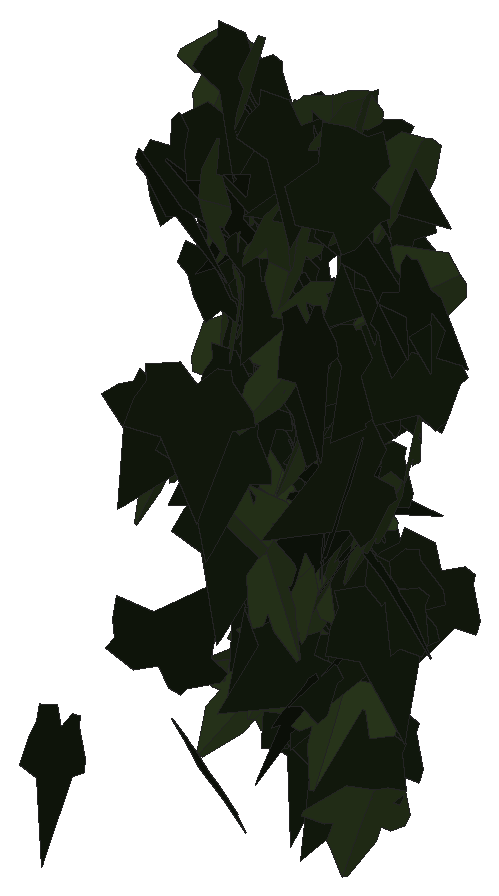
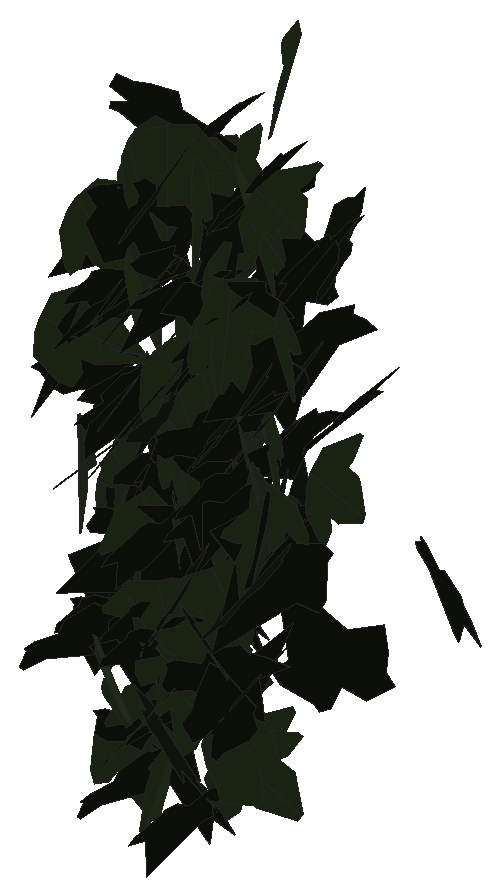
# SketchUp Ruby script. Lengths in inches.
U = 1.inch
M = Sketchup.active_model
def pt(a) = Geom::Point3d.new(a.map { |v| v * U })
def face(e, loops, mat)
  f = e.add_face(loops[0].map { |a| pt(a) })
  loops[1..].each { |l| e.add_face(l.map { |a| pt(a) }).erase! }
  f.material = f.back_material = mat if mat
  f
end
# faces: each face lists its corners as indices into pts; further lists are holes
def faces(e, pts, list, mat = nil) = list.each { |f| face(e, (f[0].is_a?(Array) ? f : [f]).map { |l| l.map { |i| pts[i] } }, mat) }
# xy, xz, yz: faces in a plane at the given z, y or x. An outline is a flat list of corners, or four numbers for a rectangle; further outlines are holes
def ring(l) = l.size == 4 ? [[l[0], l[1]], [l[2], l[1]], [l[2], l[3]], [l[0], l[3]]] : l.each_slice(2).to_a
def flat(e, list, mat, &to3) = list.each { |f| face(e, (f[0].is_a?(Array) ? f : [f]).map { |l| ring(l).map { |u, v| to3.(u, v) } }, mat) }
def xy(e, z, list, mat = nil) = flat(e, list, mat) { |x, y| [x, y, z] }
def xz(e, y, list, mat = nil) = flat(e, list, mat) { |x, z| [x, y, z] }
def yz(e, x, list, mat = nil) = flat(e, list, mat) { |y, z| [x, y, z] }
def lines(e, pts, list) = list.each { |a, b| e.add_line(pt(pts[a]), pt(pts[b])) }
# prism: a flat outline (further loops are holes) pulled along v
def prism(e, loops, v, mat = nil)
  f = face(e, loops, mat); d = Geom::Vector3d.new(v.map { |x| x * U })
  f.pushpull(f.normal.samedirection?(d) ? d.length : -d.length)
end
def box(e, o, s, mat = nil) = prism(e, [[o, [o[0] + s[0], o[1], o[2]], [o[0] + s[0], o[1] + s[1], o[2]], [o[0], o[1] + s[1], o[2]]]], [0, 0, s[2]], mat)
def at(x, y, z, deg = 0) = Geom::Transformation.translation(pt([x, y, z])) * Geom::Transformation.rotation(ORIGIN, Z_AXIS, deg.degrees)
def axes(o, x, y, z) = Geom::Transformation.new([*x, 0, *y, 0, *z, 0, *pt(o).to_a, 1])
def part(name) = M.definitions.add(name)
# library, detail: a bought-in or finely detailed component or shape, given as its bounding box
def library(name, o, s) = part(name).tap { |d| box(d.entities, o, s) }
def detail(e, o, s) = box(e.add_group.entities, o, s)
def put(e, d, t, mat = nil) = e.add_instance(d, t).tap { |i| i.material = mat if mat }
def group(e, t, mat = nil) = e.add_group.tap { |g| g.transformation = t; g.material = mat if mat }.entities
root = M.entities
M.materials.add("efeu1").color = [18, 25, 13]
M.materials.add("efeu2").color = [43, 57, 29]
c1 = part("ivyleaf_9")
p = [[1.54,2.16,1.25],[1.36,2.04,1.19],[-0.21,0.99,0.68],[-0.71,1.11,0.82],[-0.85,0.86,0.67],[-0.8,0.17,0.21],
  [-0.9,-0.01,0.1],[-0.67,-0.16,-0.02],[-0.08,-0.08,-0.05],[-0.03,-0.6,-0.4],[0.65,-0.88,-0.66],[0.83,-0.6,-0.49],
  [1.29,-0.42,-0.43],[1.8125,-0.07,-0.26],[1.21,0.44,0.15]]
faces(c1.entities,p,[[0,1,2,3,4,5,6,7,8,9,10,11,12,13,14]],"efeu1")
c2 = part("ivyleaf_10")
p = [[0,0.5,-0.03],[-0.0625,2.02,-0.43],[-0.19,2.01,-0.46],[-0.54,1.05,-0.29],[-0.52,0.625,-0.18],[-0.83,0.76,-0.28],
  [-1.16,0.64,-0.33],[-1.15,0.33,-0.24],[-0.77,-0.39,0.02],[-0.3,-0.51,0.16],[0.04,-0.48,0.23],[-0.02,2.01,-0.4375],
  [-0.06,2.01,-0.43],[0.04,-0.49,0.23],[0.67,-0.49,0.14],[1.38,0.36,-0.2],[1.375,0.51,-0.24],[0.81,0.65,-0.19],
  [0.62,0.59,-0.15],[0.6,1.09,-0.28],[0.5,1.23,-0.31]]
faces(c2.entities,p,[[0,1,2,3,4,5,6,7,8,9,10],[11,12,0,13,14,15,16,17,18,19,20]],"efeu2")
put(root,c1,axes([33.67,221.12,240.87],[0.24881,-0.31359,-0.29959],[-0.11159,0.28747,-0.39359],[0.41909,0.26272,0.07306]))
put(root,c2,axes([33.84,221.94,241.72],[-0.14855,-0.34133,0.3338],[0.13113,-0.36531,-0.3152],[0.45906,-0.0061,0.19806]))
put(root,c1,axes([33.71,221.62,239.37],[0.33206,-0.2948,-0.22985],[-0.12761,0.19957,-0.44032],[0.35136,0.35109,0.0573]))
put(root,c2,axes([33.86,221.83,237.71],[0.02125,0.46143,0.19138],[-0.03249,0.19243,-0.46034],[-0.49849,0.00713,0.03816]))
put(root,c1,axes([33.8,221.57,237.23],[0.3517,0.34567,0.0826],[0.0606,0.05617,-0.49312],[-0.3502,0.35687,-0.00239]))
put(root,c2,axes([33.73,222.03,238.11],[0.4631,-0.07129,0.17451],[0.17295,-0.02344,-0.46855],[0.07499,0.49434,0.00295]))
put(root,c1,axes([34.03,221.78,237.21],[-0.03521,-0.25322,0.4297],[0.05923,0.4256,0.25565],[-0.49523,0.0689,0.00003]))
put(root,c1,axes([33.69,220.79,240.79],[0.39813,-0.29674,-0.05863],[-0.04686,0.03523,-0.49655],[0.29882,0.40088,0.00024]))
put(root,c2,axes([34.01,221.74,238.85],[0.3219,-0.34092,-0.17364],[-0.07662,0.16488,-0.46577],[0.37485,0.32647,0.05391]))
put(root,c1,axes([33.95,221.53,239.51],[0.13311,0.29585,0.38047],[0.14222,0.35302,-0.32427],[-0.46049,0.19455,0.00983]))
put(root,c2,axes([34.02,221.64,240.13],[0.39959,-0.27835,-0.11337],[-0.07661,0.08805,-0.48619],[0.29062,0.40592,0.02772]))
put(root,c1,axes([33.78,222.41,236.97],[0.08675,-0.46042,0.17462],[0.09826,-0.15755,-0.46424],[0.48251,0.11486,0.06315]))
put(root,c2,axes([34.09,222.25,240.49],[-0.09036,-0.46837,-0.14987],[0.03951,0.14498,-0.47689],[0.49018,-0.09802,0.01081]))
put(root,c2,axes([34.34,221.37,240.95],[-0.02494,0.0348,-0.49816],[-0.30843,0.39121,0.04276],[0.39275,0.30943,0.00195]))
put(root,c2,axes([34.13,222.37,240.24],[-0.10915,-0.48793,0.00331],[-0.00759,-0.00169,-0.49994],[0.48788,-0.10919,-0.00703]))
put(root,c2,axes([34.1,222.04,238.9375],[0.24128,-0.4351,-0.04975],[-0.01733,0.04727,-0.49746],[0.43759,0.24178,0.00773]))
put(root,c2,axes([34.04,220.7,237.56],[0.04288,-0.34592,0.35847],[0.11089,-0.34414,-0.34536],[0.48566,0.10912,0.04721]))
put(root,c1,axes([33.85,222.53,239.25],[0.14288,-0.45493,0.1504],[0.05765,-0.13948,-0.47668],[0.47567,0.15356,0.0126]))
put(root,c1,axes([33.97,222.36,239],[0.00277,-0.49786,0.04616],[0.00535,-0.04612,-0.49784],[0.49996,0.00325,0.00508]))
put(root,c1,axes([34.16,221.68,236.9],[-0.18754,-0.24831,0.39137],[-0.06091,-0.40532,-0.28636],[0.45947,-0.15509,0.12178]))
put(root,c1,axes([34.25,222.34,235.14],[0.02189,0.02652,0.49882],[-0.30477,-0.39489,0.03437],[0.39578,-0.30555,-0.00112]))
put(root,c1,axes([33.91,221.24,240.2],[0.48453,0.02298,-0.12125],[0.1157,0.08626,0.47872],[0.04291,-0.49197,0.07827]))
put(root,c1,axes([34.08,222.31,238.35],[0.06115,-0.471,-0.15626],[-0.03451,0.15302,-0.47476],[0.49505,0.06885,-0.01379]))
put(root,c1,axes([34.125,221.94,241.75],[-0.0174,-0.47626,0.15125],[0.00198,-0.1514,-0.47652],[0.49969,-0.01598,0.00715]))
put(root,c1,axes([34.32,222.42,235.94],[-0.35277,-0.35374,-0.02045],[0.01422,0.01471,-0.49958],[0.35405,-0.35306,-0.00031]))
put(root,c1,axes([34.08,220.38,234.92],[-0.2088,-0.06429,0.44975],[0.43968,-0.15321,0.18222],[0.11438,0.47159,0.12051]))
put(root,c2,axes([34.42,221.91,234.4375],[-0.12256,-0.10711,-0.47276],[-0.17786,-0.44369,0.14664],[-0.45094,0.20412,0.07066]))
put(root,c1,axes([34.25,220.24,238.06],[-0.12636,-0.39607,0.27779],[0.00685,-0.28854,-0.40829],[0.48372,-0.09938,0.07834]))
put(root,c2,axes([34.23,221.83,241.89],[0.23145,-0.33891,0.2856],[0.16877,-0.23053,-0.41033],[0.40982,0.28634,0.00768]))
put(root,c1,axes([34.16,222.32,240.29],[0.14935,-0.44328,-0.17661],[-0.03479,0.17445,-0.46729],[0.4759,0.15187,0.02127]))
put(root,c2,axes([34.53,221.55,234.26],[-0.2262,-0.27985,0.34716],[-0.11696,-0.33841,-0.349],[0.4303,-0.23909,0.08763]))
put(root,c1,axes([34.33,222.23,240.5],[-0.27886,-0.36598,-0.1957],[0.11708,0.15682,-0.46011],[0.39816,-0.30244,-0.00176]))
put(root,c2,axes([34.39,222.08,240.61],[0.08881,-0.4533,0.19139],[0.06306,-0.1824,-0.46125],[0.48799,0.10607,0.02478]))
put(root,c1,axes([34.3,222.01,235.21],[-0.07086,-0.38284,0.31371],[0.0018,-0.3171,-0.38658],[0.49495,-0.05366,0.04632]))
put(root,c1,axes([34.27,222.16,237.86],[0.00646,-0.46997,-0.17053],[0.01876,0.17066,-0.4696],[0.49961,-0.00034,0.01984]))
put(root,c1,axes([34.48,222.41,238.86],[-0.24455,-0.43378,0.04507],[-0.01879,-0.04115,-0.49795],[0.43571,-0.24524,0.00382]))
put(root,c2,axes([34.5,221.97,236.74],[0.30758,0.36216,-0.15568],[-0.11657,-0.10507,-0.47473],[-0.37657,0.32833,0.0198]))
put(root,c1,axes([34.33,221.29,241.375],[0.1074,-0.44914,-0.19166],[0.00311,0.19687,-0.4596],[0.48832,0.09753,0.04508]))
put(root,c1,axes([34.48,218.11,235.15],[-0.33467,-0.02194,-0.37083],[0.37142,-0.01103,-0.33455],[0.0065,-0.4994,0.02368]))
put(root,c1,axes([34.375,221.55,238.03],[0.06981,-0.48323,0.10779],[0.02489,-0.10529,-0.48815],[0.49448,0.07352,0.00935]))
put(root,c1,axes([34.71,222.23,236.35],[-0.43102,0.0832,-0.23938],[0.22506,-0.09143,-0.43702],[-0.11649,-0.48448,0.04137]))
put(root,c2,axes([34.54,221.97,235.88],[0.19834,0.3335,0.31534],[0.15724,0.27336,-0.388],[-0.4312,0.25308,0.00356]))
put(root,c1,axes([34.37,221.84,240.88],[0.1532,-0.2372,0.41263],[0.27817,-0.30712,-0.27982],[0.3862,0.3153,0.03786]))
put(root,c1,axes([34.53,222.12,239.72],[0.21342,-0.44198,-0.09541],[-0.0301,0.09138,-0.49066],[0.45116,0.21518,0.01239]))
put(root,c1,axes([34.6875,221.82,239.51],[-0.10889,-0.43349,0.22412],[-0.02281,-0.22486,-0.446],[0.48746,-0.10736,0.02919]))
put(root,c1,axes([34.7,220.72,237.84],[-0.07293,-0.49313,0.03873],[-0.00858,-0.03788,-0.49849],[0.49458,-0.07337,-0.00293]))
put(root,c2,axes([34.93,221.63,234.95],[-0.23159,-0.35995,0.25846],[-0.04382,-0.2716,-0.41751],[0.44096,-0.21603,0.09426]))
put(root,c1,axes([34.59,222.31,240.5625],[0.11709,-0.39469,-0.28375],[0.07019,0.30253,-0.39185],[0.481,0.05193,0.12625]))
put(root,c1,axes([34.79,220.875,236.71],[-0.07808,-0.48757,0.07862],[0.00169,-0.07986,-0.49358],[0.49386,-0.07681,0.01412]))
put(root,c1,axes([34.71,222.23,233.93],[0.0721,-0.45946,-0.18358],[0.02045,0.18813,-0.46281],[0.49435,0.05923,0.04592]))
put(root,c1,axes([35.04,222.48,235.0625],[-0.42568,0.12508,-0.23054],[0.20888,-0.10412,-0.44219],[-0.15862,-0.47277,0.03639]))
put(root,c1,axes([34.81,222.4375,236.47],[-0.02774,-0.2867,0.4087],[0.04341,-0.40917,-0.28408],[0.49734,0.01972,0.0476]))
put(root,c2,axes([35.09,221.51,238.57],[-0.15771,-0.29364,0.3727],[-0.05028,-0.38019,-0.32082],[0.4718,-0.13867,0.09039]))
put(root,c2,axes([35,221.63,240.12],[-0.06515,-0.47107,0.15444],[0.06756,-0.16275,-0.46792],[0.49111,-0.0401,0.08485]))
put(root,c2,axes([35.03,222.06,238.41],[0.07731,-0.4938,0.01362],[0.00236,-0.01342,-0.49981],[0.49398,0.07734,0.00026]))
put(root,c2,axes([34.875,220.7,236.94],[-0.39341,-0.06862,-0.30086],[0.29444,0.06242,-0.39926],[0.09235,-0.49132,-0.0087]))
put(root,c1,axes([34.94,219.92,238.83],[-0.13268,-0.46122,-0.14025],[0.04085,0.13419,-0.47992],[0.48034,-0.13881,0.00207]))
put(root,c2,axes([35.04,221.875,237.64],[-0.09652,0.24725,-0.42374],[-0.02274,-0.43365,-0.24785],[-0.49007,-0.02857,0.09496]))
put(root,c2,axes([35.04,222.28,236.51],[0.41964,0.26738,-0.04911],[-0.04594,-0.01928,-0.49751],[-0.26794,0.42206,0.00839]))
put(root,c1,axes([35,222.17,238.14],[-0.23125,-0.40765,-0.17419],[0.09973,0.14359,-0.46844],[0.43195,-0.2514,0.0149]))
put(root,c2,axes([35.23,221.88,235.81],[-0.21722,-0.41649,0.17132],[-0.0816,-0.15066,-0.46973],[0.4429,-0.23203,-0.00252]))
put(root,c2,axes([35.14,221.57,241.36],[0.34943,-0.30148,-0.19237],[-0.03817,0.23598,-0.43915],[0.35558,0.3216,0.1419]))
put(root,c2,axes([35.18,221.93,239.19],[-0.12123,-0.47126,0.11496],[0.01147,-0.12125,-0.48494],[0.48495,-0.11494,0.04021]))
put(root,c1,axes([35.23,221.08,236.06],[-0.45344,0.00326,-0.21067],[0.21056,-0.01091,-0.45337],[-0.00756,-0.49987,0.00852]))
put(root,c1,axes([34.99,222.38,237.43],[0.09715,-0.4501,-0.19486],[-0.00673,0.19741,-0.45933],[0.49043,0.09187,0.0323]))
put(root,c1,axes([34.94,222.23,238.99],[0.30198,-0.39742,0.02945],[0.01542,-0.02527,-0.49912],[0.39821,0.30236,-0.00301]))
put(root,c1,axes([35.07,222.3,236.04],[-0.0495,-0.47321,-0.15371],[0.03016,0.15133,-0.47559],[0.49663,-0.05636,0.01356]))
put(root,c1,axes([35.2,221.79,234],[-0.38923,-0.09532,-0.29902],[0.30272,0.01171,-0.39778],[0.08283,-0.49069,0.0486]))
put(root,c2,axes([35.24,222.02,234.24],[-0.35114,0.34953,-0.06732],[0.04605,-0.04917,-0.49544],[-0.35296,-0.35414,0.00234]))
put(root,c1,axes([35.16,222.21,236.3125],[0.00964,-0.47305,-0.16165],[0.00515,0.16176,-0.47308],[0.49988,0.00746,0.00799]))
put(root,c1,axes([35.26,221.99,234.79],[-0.16072,-0.4301,0.19793],[0.02172,-0.21551,-0.45065],[0.47296,-0.13626,0.08796]))
put(root,c1,axes([35.15,222.19,238.99],[0.29398,-0.34073,-0.21789],[-0.09024,0.20732,-0.44595],[0.39425,0.30153,0.0604]))
put(root,c2,axes([35.41,221.74,241.73],[-0.32055,-0.38371,-0.00324],[0.0054,-0.00029,-0.49997],[0.38369,-0.32057,0.00433]))
put(root,c1,axes([35.17,222.57,234.91],[-0.00415,-0.44434,0.22922],[0.04202,-0.22873,-0.44263],[0.49821,0.01559,0.03924]))
put(root,c2,axes([35.375,222.06,236.43],[0.03789,-0.45257,0.20916],[0.0416,-0.20616,-0.45362],[0.49682,0.05178,0.02203]))
put(root,c2,axes([35.4,222.1,237.43],[0.17328,0.42078,-0.20717],[-0.11834,-0.17448,-0.45338],[-0.45384,0.20616,0.03912]))
put(root,c2,axes([35.5625,220.91,236.28],[0.36338,-0.19438,-0.28315],[-0.2552,0.12305,-0.41199],[0.22984,0.44393,-0.00978]))
put(root,c1,axes([35.26,221.71,238.125],[0.24245,-0.32511,-0.29245],[-0.1336,0.26333,-0.4035],[0.41638,0.27379,0.04082]))
put(root,c2,axes([35.47,222.16,240.39],[0.15944,-0.47146,0.04796],[0.00945,-0.04743,-0.49766],[0.4738,0.1596,-0.00622]))
put(root,c2,axes([35.66,219.26,241.75],[-0.17662,0.19426,0.42552],[-0.2642,0.33392,-0.2621],[-0.38601,-0.31743,-0.0153]))
put(root,c1,axes([35.21,221.74,236.89],[0.40309,0.14563,0.2575],[0.23109,0.11672,-0.42775],[-0.1847,0.46386,0.02679]))
put(root,c2,axes([35.62,221.56,235.71],[-0.07463,0.44496,-0.21551],[-0.08092,0.20402,0.44925],[0.48773,0.10194,0.04156]))
put(root,c1,axes([35.26,222.04,241.46],[0.2717,-0.4188,-0.02797],[-0.01249,0.02524,-0.49921],[0.41955,0.27197,0.00325]))
put(root,c1,axes([35.54,222.15,237.26],[-0.36526,-0.32631,-0.10051],[0.10528,0.03238,-0.48772],[0.3248,-0.37745,0.04506]))
put(root,c1,axes([35.375,221.2,241.6875],[-0.03275,-0.48553,0.11485],[0.05107,-0.11776,-0.48324],[0.49631,-0.01993,0.05731]))
put(root,c2,axes([35.61,220.6,241.02],[0.00458,-0.47451,-0.15753],[0.02752,0.15754,-0.47373],[0.49922,-0.00433,0.02756]))
put(root,c2,axes([35.625,221.86,241.68],[0.02651,-0.4929,0.07969],[0.01053,-0.07924,-0.49357],[0.49919,0.02784,0.00618]))
put(root,c1,axes([35.42,221.61,237.45],[-0.14077,0.0397,-0.47813],[0.45834,-0.13615,-0.14625],[-0.1418,-0.47947,0.00194]))
put(root,c2,axes([35.5625,221.66,235.94],[-0.05043,0.12651,-0.48109],[-0.00535,-0.48367,-0.12663],[-0.49742,-0.00762,0.05014]))
put(root,c1,axes([35.72,221.16,236.85],[-0.10888,0.285,-0.39613],[0.14702,-0.36786,-0.30507],[-0.46533,-0.18291,-0.0037]))
put(root,c1,axes([35.41,222.17,240.07],[0.12234,-0.46436,0.13928],[0.05037,-0.1307,-0.47998],[0.48218,0.13147,0.0148]))
put(root,c1,axes([35.4,222,241.1],[0.03024,-0.1364,-0.48008],[0.15018,0.46116,-0.12156],[0.47595,-0.13685,0.06886]))
put(root,c1,axes([35.75,220.91,235.34],[-0.27378,-0.26816,0.32114],[-0.0996,-0.33098,-0.36129],[0.40635,-0.26181,0.12782]))
put(root,c1,axes([35.5,222.01,238.92],[0.03588,-0.36332,-0.34163],[0.04813,0.34343,-0.36019],[0.49638,-0.00704,0.05962]))
put(root,c1,axes([35.56,222.3,240.39],[-0.08236,-0.46986,-0.14984],[0.04637,0.14386,-0.47661],[0.49098,-0.09241,0.01988]))
put(root,c1,axes([35.73,222.375,238.76],[-0.20117,-0.34645,0.29917],[-0.09931,-0.28596,-0.39795],[0.44684,-0.21953,0.04624]))
put(root,c2,axes([35.87,221.74,237.85],[-0.13794,0.30562,0.3709],[-0.22907,0.29741,-0.33026],[-0.42249,-0.26104,0.05797]))
put(root,c1,axes([35.87,220.87,235.05],[-0.22516,0.33865,-0.29089],[0.14383,-0.2534,-0.40633],[-0.42263,-0.26666,0.0167]))
put(root,c1,axes([35.71,222.25,233.92],[-0.14302,-0.45127,0.16094],[-0.01873,-0.16256,-0.47246],[0.47874,-0.14118,0.02959]))
put(root,c1,axes([35.78,222.34,239.77],[-0.24516,-0.34132,0.27092],[-0.02863,-0.29756,-0.40079],[0.43483,-0.21203,0.12636]))
put(root,c1,axes([35.72,222.71,238.13],[-0.15583,-0.39606,0.2624],[0.03731,-0.28551,-0.40877],[0.47363,-0.10782,0.11853]))
put(root,c2,axes([35.87,221.31,234.64],[0.26852,0.38425,-0.17393],[-0.09215,-0.14776,-0.4687],[-0.41159,0.28377,-0.00854]))
put(root,c2,axes([35.96,222.43,241.02],[-0.08505,-0.42365,0.25157],[0.03985,-0.26037,-0.42499],[0.4911,-0.05224,0.07805]))
put(root,c1,axes([35.72,222.03,240.11],[0.2105,-0.44954,0.05999],[0.02518,-0.05445,-0.49639],[0.45283,0.212,-0.00028]))
put(root,c1,axes([35.87,221.92,238.53],[-0.07523,-0.34079,0.35805],[-0.01409,-0.36055,-0.34613],[0.49411,-0.06217,0.04464]))
put(root,c1,axes([35.8125,220.78,239.51],[-0.23219,-0.03456,-0.44147],[0.43964,0.04163,-0.23449],[0.05296,-0.49706,0.01105]))
put(root,c1,axes([36.1,221.85,235.82],[-0.40737,-0.28796,-0.03364],[0.02782,0.01893,-0.49887],[0.28858,-0.40831,0.0006]))
put(root,c1,axes([35.92,222,235.99],[-0.13048,-0.45253,-0.16791],[0.05052,0.16018,-0.47095],[0.48002,-0.13986,0.00392]))
put(root,c1,axes([35.84,222.31,239.93],[0.14391,-0.47287,-0.07542],[-0.01362,0.07468,-0.4942],[0.47865,0.14429,0.00861]))
put(root,c2,axes([35.8125,222.08,234.8],[0.27308,-0.3022,-0.29001],[0.23121,-0.17991,0.40519],[-0.34924,-0.3554,0.04149]))
put(root,c2,axes([36.28,222.49,239.52],[-0.08227,-0.19845,0.4515],[-0.21028,-0.39993,-0.2141],[0.44611,-0.22511,-0.01765]))
put(root,c1,axes([36.16,221.36,234.1875],[-0.39926,-0.29878,-0.03638],[0.02472,0.02768,-0.49862],[0.29997,-0.39995,-0.00733]))
put(root,c2,axes([35.81,220.11,236.73],[0.29624,-0.07357,0.39602],[0.38896,-0.07548,-0.30498],[0.10466,0.48876,0.01251]))
put(root,c1,axes([36.35,221.12,236.99],[-0.24196,0.43252,-0.06616],[0.03227,-0.05776,-0.4956],[-0.43636,-0.24411,0.00004]))
put(root,c2,axes([36.26,222.15,237.99],[0.22089,-0.37068,-0.25259],[-0.0564,0.25637,-0.42555],[0.445,0.21649,0.07144]))
put(root,c1,axes([36.5,221,237.81],[-0.48634,-0.00257,0.11606],[-0.11606,-0.00126,-0.48634],[0.00279,-0.49999,0.00063]))
put(root,c1,axes([36.57,220.87,241.53],[-0.42952,0.02481,0.25475],[-0.25516,-0.00246,-0.42998],[-0.02008,-0.49938,0.01478]))
put(root,c1,axes([36.19,222.61,235.77],[-0.17409,-0.45444,0.1148],[-0.02135,-0.11464,-0.48621],[0.46823,-0.17419,0.02052]))
put(root,c1,axes([36.03,218.76,234.94],[0.40499,-0.23122,-0.18032],[0.17189,-0.0619,0.46543],[-0.23756,-0.43898,0.02935]))
put(root,c1,axes([36.12,221.72,235.67],[0.02552,-0.4846,-0.12047],[0.00443,0.12084,-0.48516],[0.49933,0.0237,0.01046]))
put(root,c2,axes([36.24,221.65,237.14],[0.09695,-0.32994,0.36296],[0.10447,-0.3476,-0.34388],[0.47925,0.14252,0.00154]))
put(root,c1,axes([36.51,222.08,238.81],[-0.43973,-0.18605,0.14839],[-0.13244,-0.0677,-0.47736],[0.19772,-0.45913,0.01026]))
put(root,c1,axes([36.56,220.47,237.74],[-0.15658,0.07592,-0.46874],[-0.41412,0.21968,0.17392],[0.23235,0.44269,-0.00591]))
put(root,c1,axes([36.25,221.91,239.61],[0.17603,-0.20516,-0.42062],[-0.23485,0.34998,-0.26899],[0.40479,0.29227,0.02685]))
put(root,c1,axes([36.02,221.8,236.1875],[0.23683,-0.33801,0.28224],[0.16676,-0.22776,-0.41269],[0.40755,0.28961,0.00486]))
put(root,c2,axes([36.49,221,233.7],[-0.26278,-0.40805,0.12015],[-0.06844,-0.09883,-0.48533],[0.41983,-0.27152,-0.00391]))
